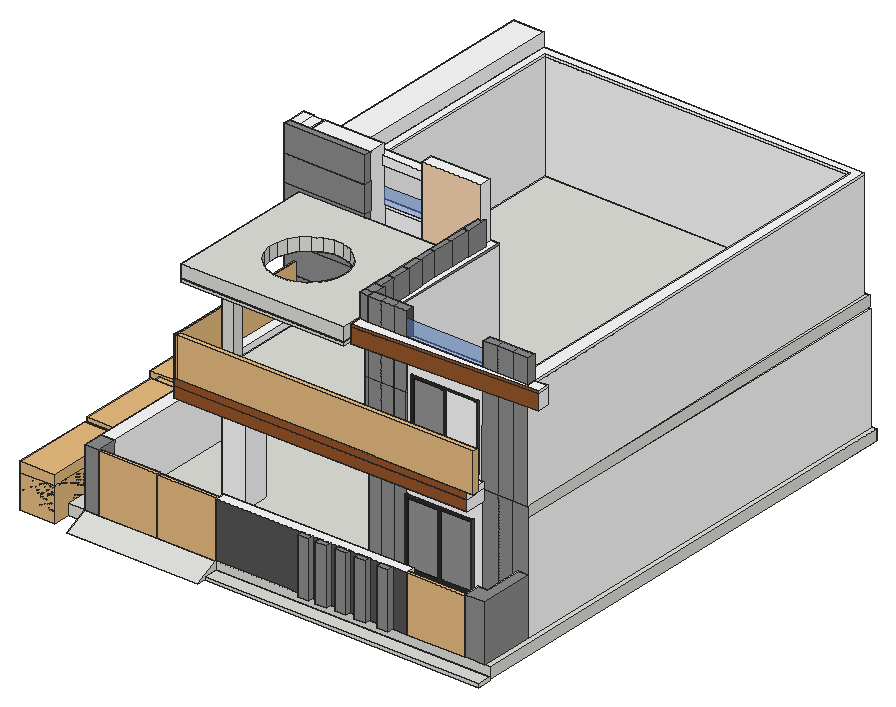
# SketchUp Ruby script. Lengths in inches.
U = 1.inch
M = Sketchup.active_model
def pt(a) = Geom::Point3d.new(a.map { |v| v * U })
def face(e, loops, mat)
  f = e.add_face(loops[0].map { |a| pt(a) })
  loops[1..].each { |l| e.add_face(l.map { |a| pt(a) }).erase! }
  f.material = f.back_material = mat if mat
  f
end
# faces: each face lists its corners as indices into pts; further lists are holes
def faces(e, pts, list, mat = nil) = list.each { |f| face(e, (f[0].is_a?(Array) ? f : [f]).map { |l| l.map { |i| pts[i] } }, mat) }
# xy, xz, yz: faces in a plane at the given z, y or x. An outline is a flat list of corners, or four numbers for a rectangle; further outlines are holes
def ring(l) = l.size == 4 ? [[l[0], l[1]], [l[2], l[1]], [l[2], l[3]], [l[0], l[3]]] : l.each_slice(2).to_a
def flat(e, list, mat, &to3) = list.each { |f| face(e, (f[0].is_a?(Array) ? f : [f]).map { |l| ring(l).map { |u, v| to3.(u, v) } }, mat) }
def xy(e, z, list, mat = nil) = flat(e, list, mat) { |x, y| [x, y, z] }
def xz(e, y, list, mat = nil) = flat(e, list, mat) { |x, z| [x, y, z] }
def yz(e, x, list, mat = nil) = flat(e, list, mat) { |y, z| [x, y, z] }
def lines(e, pts, list) = list.each { |a, b| e.add_line(pt(pts[a]), pt(pts[b])) }
# prism: a flat outline (further loops are holes) pulled along v
def prism(e, loops, v, mat = nil)
  f = face(e, loops, mat); d = Geom::Vector3d.new(v.map { |x| x * U })
  f.pushpull(f.normal.samedirection?(d) ? d.length : -d.length)
end
def box(e, o, s, mat = nil) = prism(e, [[o, [o[0] + s[0], o[1], o[2]], [o[0] + s[0], o[1] + s[1], o[2]], [o[0], o[1] + s[1], o[2]]]], [0, 0, s[2]], mat)
def at(x, y, z, deg = 0) = Geom::Transformation.translation(pt([x, y, z])) * Geom::Transformation.rotation(ORIGIN, Z_AXIS, deg.degrees)
def axes(o, x, y, z) = Geom::Transformation.new([*x, 0, *y, 0, *z, 0, *pt(o).to_a, 1])
def part(name) = M.definitions.add(name)
# library, detail: a bought-in or finely detailed component or shape, given as its bounding box
def library(name, o, s) = part(name).tap { |d| box(d.entities, o, s) }
def detail(e, o, s) = box(e.add_group.entities, o, s)
def put(e, d, t, mat = nil) = e.add_instance(d, t).tap { |i| i.material = mat if mat }
def group(e, t, mat = nil) = e.add_group.tap { |g| g.transformation = t; g.material = mat if mat }.entities
root = M.entities
M.materials.add("Glass_Tinted_Gray").color = [0, 0, 0]
M.materials["Glass_Tinted_Gray"].alpha = 0.125
M.materials.add("[0135_DarkGray]").color = [81, 81, 81]
M.materials.add("[Color C03]").color = [255, 218, 181]
M.materials.add("[Color M00]").color = [255, 255, 255]
M.materials.add("[Color M04]").color = [142, 142, 142]
M.materials.add("[Color M06]").color = [86, 86, 86]
M.materials.add("[Mirror 02]").color = [229, 229, 229]
M.materials.add("[Terrazzo Light Blue]").color = [196, 214, 227]
M.materials.add("[Translucent Glass Blue]").color = [100, 149, 237]
M.materials["[Translucent Glass Blue]"].alpha = 0.5
M.materials.add("[Wood Cherry Original]").color = [152, 86, 42]
c1 = part("PENTEK_RP Fineline 50S_Sliding_DoorCase_E1")
box(c1.entities,[0,0,0],[1.51,3.66,99.27],"[0135_DarkGray]")
c2 = part("PENTEK_RP Fineline 50S_SlidingDooe_Case_E2")
box(c2.entities,[0,0,0],[96.25,3.66,1.51],"[0135_DarkGray]")
c3 = part("pentek_RP Fineline 50S_SlidingDoor_Case")
put(c3.entities,c1,at(97.76,0,0))
put(c3.entities,c2,at(1.51,0,0))
put(c3.entities,c1,at(0,0,0))
put(c3.entities,c2,at(1.51,0,97.76))
c4 = part("PENTEK_RP Fineline 50S_SlidingDoor_GlazingBead_2")
box(c4.entities,[0,0,0],[0.56,0.59,94.39],"[0135_DarkGray]")
c5 = part("PENTEK_RP Fineline 50S_SlidingDoor_Glass")
box(c5.entities,[0,0,0],[46.58,0.16,94.39],"Glass_Tinted_Gray")
c6 = part("PENTEK_RP Fineline 50S_SlidingDoor_GlazingBead")
box(c6.entities,[0,0,0],[45.47,0.59,0.56],"[0135_DarkGray]")
c7 = part("PENTEK_RP Fineline 50S_SlidingDoor_Leaf_E1")
xy(c7.entities,0,[[0,0,0.93,1.97],[0.93,1.57,1.49,1.97]],"[0135_DarkGray]")
xy(c7.entities,96.25,[[0,0,0.93,0,0.93,1.57,1.49,1.57,1.49,1.97,0,1.97]],"[0135_DarkGray]")
xz(c7.entities,0,[[0,0,0.93,96.25]],"[0135_DarkGray]")
xz(c7.entities,1.57,[[0.93,0,1.49,95.32],[0.93,95.32,1.49,96.25]],"[0135_DarkGray]")
xz(c7.entities,1.97,[[0,0,1.49,96.25]],"[0135_DarkGray]")
yz(c7.entities,0,[[0,0,1.97,96.25]],"[0135_DarkGray]")
yz(c7.entities,0.93,[[0,0,1.57,0.93],[0,0.93,1.57,95.32],[0,95.32,1.57,96.25]],"[0135_DarkGray]")
yz(c7.entities,1.49,[[1.57,0,1.97,95.32],[1.57,95.32,1.97,96.25]],"[0135_DarkGray]")
c8 = part("PENTEK_RP Fineline 50S_SlidingDoor_Leaf_E2")
xy(c8.entities,0,[[0,0,0,1.57,0.56,1.57,0.56,1.97,46.02,1.97,46.02,1.57,46.58,1.57,46.58,0]],"[0135_DarkGray]")
xy(c8.entities,0.93,[[0,0,46.58,1.57]],"[0135_DarkGray]")
xy(c8.entities,1.49,[[0.56,1.57,46.02,1.97]],"[0135_DarkGray]")
xz(c8.entities,0,[[0,0,46.58,0.93]],"[0135_DarkGray]")
xz(c8.entities,1.57,[[0,0,0.56,0.93],[46.02,0,46.58,0.93],[0.56,0.93,46.02,1.49]],"[0135_DarkGray]")
xz(c8.entities,1.97,[[0.56,0,46.02,1.49]],"[0135_DarkGray]")
yz(c8.entities,0,[[0,0,1.57,0.93]],"[0135_DarkGray]")
yz(c8.entities,0.56,[[1.57,0,1.97,0.93],[1.57,0.93,1.97,1.49]],"[0135_DarkGray]")
yz(c8.entities,46.02,[[1.57,0,1.97,0.93],[1.57,0.93,1.97,1.49]],"[0135_DarkGray]")
yz(c8.entities,46.58,[[0,0,1.57,0.93]],"[0135_DarkGray]")
c9 = part("PENTEK_RP Fineline S_SlidingDoor_Leaf1")
put(c9.entities,c4,at(0.93,0,0.93))
put(c9.entities,c4,at(46.96,0,0.93))
put(c9.entities,c5,at(1.49,1.42,0.93))
put(c9.entities,c6,at(1.49,0,0.93))
put(c9.entities,c5,at(1.49,0.59,0.93),"[Terrazzo Light Blue]")
put(c9.entities,c7,at(0,0,0))
put(c9.entities,c7,axes([48.44,0,0],[-1,0,0],[0,1,0],[0,0,1]))
put(c9.entities,c8,axes([0.93,0,96.25],[1,0,0],[0,1,0],[0,0,-1]))
put(c9.entities,c8,at(0.93,0,0))
put(c9.entities,c6,at(1.49,0,94.77))
c10 = part("PENTEK_RP Fineline 50S_SlidingDoor_Leaf2")
put(c10.entities,c5,at(1.49,1.42,0.93))
put(c10.entities,c6,at(1.49,0,94.77))
put(c10.entities,c4,at(46.96,0,0.93))
put(c10.entities,c5,at(1.49,0.59,0.93),"[Mirror 02]")
put(c10.entities,c4,at(0.93,0,0.93))
put(c10.entities,c7,at(0,0,0))
put(c10.entities,c7,axes([48.44,0,0],[-1,0,0],[0,1,0],[0,0,1]))
put(c10.entities,c6,at(1.49,0,0.93))
put(c10.entities,c8,axes([0.93,0,96.25],[1,0,0],[0,1,0],[0,0,-1]))
put(c10.entities,c8,at(0.93,0,0))
c11 = part("PENTEK - Slimmest Steel Sliding Door / Window\#1")
put(c11.entities,c3,at(0,-1.88,-0.09))
put(c11.entities,c9,at(1.51,-2.27,1.42))
put(c11.entities,c10,at(49.32,-0.3,1.42))
c12 = library("door",[38.93,25.48,0],[40,9.94,82.68])
c13 = library("4",[-16.3,-15.81,0],[32.6,31.62,37.8])
c14 = library("Glass railing",[-3.84,-0.8125,0],[184.69,5.8,43.77])
c15 = library("GATE",[0,0,0],[65.3125,3.71,50.96])
c16 = library("Broadleaf shrub",[-20.25,-26.94,0.18],[38.61,38.31,37.53])
box(root,[161.95,100.9375,132],[13.31,11.6875,105.125])
xy(root,-12,[[68.78,0,215.96,24.87],[215.96,8.81,523.46,24.87]])
xy(root,-8.5,[[215.96,8.81,523.46,24.87]])
xy(root,-0.5,[[151.43,114.08,151.27,142.08,178.52,142.08,178.52,114.08]],"[Color M00]")
xy(root,0,[[68.78,24.89,84.94,47.54],[215.5625,25.71,399.99,26.76,412.56,26.83,428.17,26.92,428.11,37.92,215.5,36.71],[493.76,27.36,493.76,45.88,504.01,45.88,504.01,88.97,515.68,89.71,515.68,27.36],[68.78,47.54,84.94,47.54,84.94,542.67,155.68,542.67,155.68,569.71,68.78,569.71],[504.01,88.97,515.68,89.71,504.01,89.71],
  [[335.68,89.71,335.68,261.83,155.68,261.83,155.68,569.71,515.68,569.71,515.68,89.71],[344.68,98.71,506.68,98.71,506.68,560.71,164.68,560.71,164.68,270.83,344.68,270.83]],[344.68,98.71,506.68,98.71,506.68,560.71,164.68,560.71,164.68,270.83,344.68,270.83]],"[Color M00]")
xy(root,62.34,[[215.5625,25.71,215.5,36.71,428.11,37.92,428.17,26.92,412.56,26.83,399.99,26.76]],"[Color M00]")
xy(root,63.0625,[[493.76,27.36,515.68,27.36,515.68,89.71,504.01,88.97,504.01,45.88,493.76,45.88]],"[Color M04]")
xy(root,65.5625,[[68.78,47.54,68.78,569.71,155.68,569.71,155.68,542.67,84.94,542.67,84.94,47.54]],"[Color M00]")
xy(root,65.5625,[[68.78,24.89,84.94,47.54]],"[Color M04]")
xy(root,73.4375,[[125.21,233.58,136.89,241.14],[136.93,233.58,136.89,241.14,136.8,257.14,212.86,257.58,212.99,234.01],[125.64,241.14,125.64,260.77,136.78,260.77,136.8,257.14,136.89,241.14]],"[Color M00]")
xy(root,97.01,[[136.8,257.14,136.8,257.39,212.86,257.83,212.86,257.58]],"[Color M00]")
xy(root,119.3125,[[114.96,260.97,148.83,568.64]],"[Color M00]")
xy(root,120,[[137.9,63.43,136.93,233.58,150.74,233.66,151.27,142.08,151.27,114.08,151.43,114.08,151.58,87.63,335.96,88.68,339.22,88.7,364.71,88.85,376.84,88.92,378.17,88.92,465.72,89.42,465.86,65.3],[[335.68,89.71,515.68,89.71,515.68,569.71,155.68,569.71,155.68,261.83,335.68,261.83],[344.68,98.71,344.68,270.83,164.68,270.83,164.68,560.71,506.68,560.71,506.68,98.71]],[151.27,114.08,151.27,142.08,151.43,114.08],[151.43,114.08,178.52,114.08,178.52,142.08,151.27,142.08],[150.74,233.66,212.99,234.01,212.86,257.83,150.61,257.47],
  [136.8,257.39,136.78,260.77,136.77,261.05,150.59,261.13,150.61,257.47]],"[Color M00]")
xy(root,131.4375,[[337.83,97.64,499.83,97.64,499.83,559.64,157.83,559.64,157.83,269.77,337.83,269.77]],"[Color M00]")
xy(root,132,[[137.9,63.43,465.86,65.3,465.72,88.64,335.96,88.64,332.77,88.51,332.77,88.66,151.58,87.63,150.7,241.14,136.89,241.14],[332.77,88.51,332.77,88.66,364.71,88.85,465.72,89.42,465.72,89.38,378.17,88.88,339.22,88.66,335.96,88.64],[[465.72,88.64,465.72,89.42,364.71,88.85,332.77,88.66,332.1875,102.6,335.375,102.73,328.83,260.77,216.72,260.77,216.72,241.14,150.7,241.14,150.59,260.77,150.59,261.13,148.83,261.12,148.83,568.64,508.83,568.64,515.57,89.7,498.73,88.64],[337.83,97.64,499.83,97.64,499.83,559.64,157.83,559.64,157.83,269.77,337.83,269.77]],[335.96,88.64,339.22,88.66,378.17,88.88,465.72,89.38,465.72,89.36,339.22,88.64],[339.22,88.64,465.72,89.36,465.72,88.79,439.91,88.64],
  [439.91,88.64,465.72,88.79,465.72,88.64],[498.73,88.64,515.57,89.7,515.58,88.64],[136.89,241.14,136.89,260.77,136.78,260.77],[136.89,241.14,148.96,260.77],[148.96,241.14,150.34,260.77],
  [150.34,241.14,150.7,241.14,150.59,260.77,150.34,260.77],[263.14,255.33,270.72,260.77],[310.72,255.33,328.83,260.77],[136.78,260.77,148.83,260.77,148.83,260.97,136.77,260.97],[148.83,260.77,148.83,261.12,150.59,261.13,150.59,260.77],
  [136.77,260.97,148.83,260.97,148.83,261.12,136.77,261.05],[114.96,285.03,131.08,285.03,131.89,553.28,114.96,553.28],[131.08,285.03,148.83,285.03,148.83,553.28,131.89,553.28]],"[Color M00]")
xy(root,139.01,[[125.21,233.58,136.89,241.14]],"[Color M00]")
xy(root,139.5625,[[137.9,63.43,465.86,65.3,465.72,88.64,335.96,88.64,332.77,88.51,332.77,88.66,151.58,87.63,150.59,260.77,148.83,260.77,148.83,261.12,136.77,261.05,136.77,260.97,136.89,241.14]],"[Color M00]")
xy(root,225.26,[[270.72,255.33,310.72,260.77]],"[Color M00]")
xy(root,230.5625,[[114.96,285.03,148.83,553.28]],"[Color M00]")
xy(root,235.0625,[[326.7,76.5,319.09,260.36,328.83,260.77,335.375,102.73,332.1875,102.6,332.77,88.51,335.96,88.64,515.48,96.07,515.41,97.64,529.98,98.24,530.53,84.9375]],"[Color M00]")
xy(root,240.21,[[[142.34,68.02,324.65,233.58],[229.57,102.99,239.9375,105.52,249.29,110.64,257.01,118.01,262.55,127.13,265.55,137.37,265.79,148.04,263.26,158.41,258.13,167.77,250.76,175.48,241.64,181.02,231.4,184.02,220.73,184.26,210.37,181.73,201.01,176.61,193.29,169.23,187.75,160.12,184.76,149.875,184.52,139.21,187.04,128.84,192.17,119.48,199.54,111.77,208.66,106.22,218.9,103.23]]])
xy(root,252,[[326.7,76.5,319.09,260.36,328.83,260.77,148.83,260.77,148.83,568.64,508.83,568.64,515.46,97.64,499.83,97.64,499.83,559.64,157.83,559.64,157.83,269.77,337.83,269.77,337.83,97.64,335.58,97.64,335.96,88.64,378.93,90.42,378.93,88.64,465.05,88.64,465.05,93.99,515.48,96.07,515.41,97.64,515.46,97.64,529.98,98.24,530.53,84.9375],[378.93,88.64,465.05,88.64,465.05,93.99,378.93,90.42],[378.93,90.42,465.05,93.99,465.05,97.64,378.93,97.64]],"[Color M00]")
xy(root,254.34,[[[142.34,68.02,324.65,233.58],[229.57,102.99,218.9,103.23,208.66,106.22,199.54,111.77,192.17,119.48,187.04,128.84,184.52,139.21,184.76,149.875,187.75,160.12,193.29,169.23,201.01,176.61,210.37,181.73,220.73,184.26,231.4,184.02,241.64,181.02,250.76,175.48,258.13,167.77,263.26,158.41,265.79,148.04,265.55,137.37,262.55,127.13,257.01,118.01,249.29,110.64,239.9375,105.52]]])
xy(root,254.875,[[326.7,76.5,530.53,84.9375,529.98,98.24,515.46,97.64,515.48,96.07,465.05,93.99,465.05,88.64,378.93,88.64,378.93,90.42,335.96,88.64,335.66,95.79,335.58,97.64,335.58,95.79,335.66,95.79,335.66,88.64,326.2,88.64,326.2,109.3,325.34,109.3,326.2,88.64],[515.48,96.07,515.46,97.64,515.41,97.64],[[499.83,97.64,515.46,97.64,508.83,568.64,148.83,568.64,148.83,260.77,263.14,260.77,263.14,268.2,328.83,268.2,328.83,260.77,319.09,260.36,325.34,109.3,326.2,109.3,326.2,127.73,326.5,127.73,326.5,148.09,333.9375,148.09,333.9375,127.73,333.88,127.73,333.88,109.3,337.83,109.3,337.83,269.77,157.83,269.77,157.83,559.64,499.83,559.64],[325.7,167.61,325.7,210.94,325.6,210.94,325.6,234.09,325.43,234.09,325.43,258.07,332.24,258.07,332.24,234.09,331.91,234.09,331.91,210.94,332.06,210.94,332.06,187.3125,331.56,187.3125,331.56,167.61],[326.5,148.09,325.7,167.37,331.56,167.61,333.08,167.67,333.875,148.4]],[136.89,260.27,148.96,260.77],[150.34,260.27,216.72,260.77],
  [216.72,260.27,263.14,260.77,216.72,260.77],[263.14,260.77,328.83,268.2],[114.96,553.28,148.83,568.64]],"[Color M00]")
xy(root,269.75,[[114.96,260.97,136.77,260.97,136.77,261.05,148.83,261.12,148.83,568.64,114.96,568.64]],"[Color M00]")
xy(root,281.3125,[[326.2,88.64,335.66,95.79],[335.96,88.64,350.49,88.64,350.49,97.64,335.58,97.64,335.66,95.79],[350.49,88.64,364.71,97.64],[364.71,88.64,378.93,97.64],[465.05,88.64,480.99,97.64],
  [480.99,88.64,498.29,97.64],[498.29,88.64,515.58,88.64,515.46,97.64,498.29,97.64],[326.2,95.79,335.58,95.79,335.58,97.64,337.83,97.64,337.83,109.3,326.2,109.3],[326.2,109.3,333.88,127.73],[326.5,127.73,333.9375,148.09],
  [326.5,148.09,333.875,148.4,333.08,167.67,331.56,167.61,325.7,167.37],[325.7,167.61,331.56,187.3125],[325.7,187.3125,332.06,210.94],[325.6,210.94,331.91,234.09],[325.43,234.09,332.24,258.07]],"[Color M04]")
xy(root,297.05,[[216.72,256.41,216.72,260.27,212.1,260.27,212.1,266.91,263.14,266.91,263.14,256.41]],"[Color M00]")
xy(root,306.86,[[216.72,256.41,263.14,256.41,263.14,266.91,212.1,266.91,212.1,260.27,216.72,260.27]],"[Color M00]")
xy(root,317.125,[[125.64,241.14,136.89,260.77],[136.89,241.14,148.96,260.27],[150.34,241.14,216.72,260.27],[263.14,255.33,328.83,268.2]],"[Color M00]")
xz(root,8.81,[[215.96,-12,523.46,-8.5]])
xz(root,24.87,[[215.96,-12,523.46,-8.5]])
xz(root,24.89,[[68.78,0,84.94,65.5625]],"[Color M04]")
xz(root,27.36,[[493.76,0,515.68,63.0625]],"[Color M04]")
xz(root,45.88,[[493.76,0,504.01,63.0625]],"[Color M00]")
xz(root,47.54,[[68.78,0,84.94,65.5625]],"[Color M00]")
xz(root,68.02,[[142.34,235.59,324.65,238.96],[142.34,238.96,324.65,240.21],[142.34,240.21,324.65,254.34]])
xz(root,88.64,[[335.96,132,339.22,139.5625],[339.22,132,350.49,139.5625],[350.49,132,364.71,139.5625],[364.71,132,378.93,139.5625],[378.93,132,439.91,139.5625],
  [439.91,132,463.57,139.5625],[463.57,132,463.66,139.5625,463.57,139.5625],[378.93,139.5625,463.66,139.5625,465.05,252,378.93,252],[378.93,252,465.05,254.875]],"[Color M00]")
xz(root,88.64,[[465.72,132,481.89,132,480.99,252,465.05,252,463.66,139.5625,465.72,139.5625],[481.89,132,498.73,132,498.29,252,480.99,252],[498.73,132,515.58,132,515.58,281.3125,498.29,281.3125,498.29,252],[335.96,139.5625,350.49,281.3125],[350.49,139.5625,378.93,139.5625,378.93,252,364.71,252,364.71,281.3125,350.49,281.3125],
  [364.71,252,378.93,281.3125],[465.05,252,480.99,281.3125],[480.99,252,498.29,281.3125],[326.2,254.875,335.66,281.3125]],"[Color M04]")
xz(root,88.64,[[463.57,132,463.66,139.5625,465.72,139.5625,465.72,132]],"[Color M06]")
xz(root,88.64,[[378.93,254.875,465.05,274.03]],"[Translucent Glass Blue]")
xz(root,89.71,[[335.68,0,515.68,120]],"[Color M04]")
xz(root,95.79,[[335.58,254.875,335.66,281.3125]],"[Color M00]")
xz(root,97.64,[[337.83,131.4375,499.83,132],[335.58,252,337.83,254.875],[499.83,252,515.46,254.875],[515.41,252,515.46,254.875],[335.58,254.875,337.83,281.3125],
  [499.83,254.875,515.46,281.3125]],"[Color M00]")
xz(root,97.64,[[337.83,132,337.83,281.3125,378.93,281.3125,378.93,252,465.05,252,465.05,281.3125,499.83,281.3125,499.83,132]],"[Color M04]")
xz(root,98.71,[[344.68,0,506.68,120]],"[Color M00]")
xz(root,109.3,[[326.2,254.875,333.88,281.3125],[333.88,254.875,337.83,281.3125]],"[Color M00]")
xz(root,114.08,[[151.43,-0.5,178.52,120]],"[Color M00]")
xz(root,127.73,[[326.2,254.875,326.5,281.3125],[326.5,254.875,333.88,281.3125],[333.88,254.875,333.9375,281.3125]],"[Color M00]")
xz(root,142.08,[[151.27,-0.5,178.52,120]],"[Color M00]")
xz(root,148.09,[[326.5,254.875,333.9375,281.3125]],"[Color M00]")
xz(root,167.61,[[325.7,254.875,331.56,281.3125]],"[Color M00]")
xz(root,187.3125,[[325.7,254.875,331.56,281.3125]],"[Color M00]")
xz(root,210.94,[[325.6,254.875,325.7,281.3125],[325.7,254.875,331.91,281.3125],[331.91,254.875,332.06,281.3125]],"[Color M00]")
xz(root,233.58,[[142.34,235.59,324.65,238.96],[142.34,238.96,324.65,240.21],[142.34,240.21,324.65,254.34]])
xz(root,233.58,[[136.89,97.01,136.93,120],[136.89,97.01,136.93,120]],"[Color M00]")
xz(root,233.58,[[125.21,73.4375,136.89,97.01],[125.21,97.01,136.89,120],[125.21,120,136.89,139.01]],"[Color M04]")
xz(root,234.09,[[325.43,254.875,325.6,281.3125],[325.6,254.875,331.91,281.3125],[331.91,254.875,332.24,281.3125]],"[Color M00]")
xz(root,241.14,[[125.21,73.4375,125.64,139.01],[136.89,132,148.96,132,148.96,287.4375,136.89,287.4375,136.89,317.125,125.64,317.125,125.64,139.01,136.89,139.01],[150.34,132,216.72,287.4375],[136.89,287.4375,148.96,317.125],[148.96,287.4375,150.34,317.125]],"[Color M00]")
xz(root,255.33,[[263.14,132,270.72,132,270.72,225.26,310.72,225.26,310.72,132,328.83,132,328.83,317.125,263.14,317.125]],"[Color C03]")
xz(root,256.41,[[216.72,297.05,263.14,306.86]],"[Color M00]")
xz(root,258.07,[[325.43,254.875,332.24,281.3125]],"[Color M06]")
xz(root,260.27,[[136.89,254.875,148.96,317.125],[150.34,254.875,216.72,254.875,216.72,297.05,212.1,297.05,212.1,306.86,216.72,306.86,216.72,317.125,150.34,317.125],[212.1,297.05,216.72,306.86]],"[Color M00]")
xz(root,260.77,[[125.64,73.4375,125.64,317.125,136.89,317.125,136.89,252,148.83,252,148.83,139.5625,136.89,139.5625,136.89,132,136.78,132,136.78,73.4375],[136.89,132,148.83,139.5625],[148.83,132,148.96,139.5625],[148.96,132,150.34,139.5625],[150.34,132,150.59,139.5625],
  [216.72,132,263.14,252],[270.72,132,310.72,225.26],[148.83,139.5625,148.96,252],[148.96,139.5625,150.34,252],[136.89,252,148.83,254.875],
  [148.83,252,148.96,254.875],[148.96,252,150.34,254.875],[150.34,252,216.72,254.875],[216.72,252,263.14,254.875],[263.14,252,328.83,254.875]],"[Color M00]")
xz(root,260.97,[[114.96,119.3125,148.83,119.3125,148.83,132,136.77,132,136.77,269.75,114.96,269.75]],"[Wood Cherry Original]")
xz(root,261.83,[[155.68,0,335.68,120]],"[Color M00]")
xz(root,266.91,[[212.1,297.05,263.14,306.86]],"[Color M00]")
xz(root,268.2,[[263.14,254.875,328.83,317.125]],"[Color M00]")
xz(root,269.77,[[157.83,131.4375,337.83,132],[157.83,132,337.83,252],[157.83,252,337.83,254.875]],"[Color M00]")
xz(root,270.83,[[164.68,0,344.68,120]],"[Color M00]")
xz(root,285.03,[[114.96,132,148.83,230.5625]],"[Color M00]")
xz(root,542.67,[[84.94,0,155.68,65.5625]],"[Color M00]")
xz(root,553.28,[[114.96,132,148.83,230.5625],[114.96,230.5625,148.83,254.875]],"[Color M00]")
xz(root,559.64,[[157.83,131.4375,499.83,132],[157.83,132,499.83,252],[157.83,252,499.83,254.875]],"[Color M00]")
xz(root,560.71,[[164.68,0,506.68,120]],"[Color M00]")
xz(root,568.64,[[114.96,119.3125,148.83,254.875],[148.83,132,508.83,252],[148.83,252,508.83,254.875],[114.96,254.875,148.83,269.75]],"[Color M00]")
xz(root,569.71,[[68.78,0,155.68,65.5625],[155.68,0,515.68,120]],"[Color M00]")
yz(root,68.78,[[0,-12,24.89,0,24.87,-12]])
yz(root,68.78,[[47.54,0,569.71,65.5625]],"[Color M00]")
yz(root,68.78,[[24.89,0,47.54,65.5625]],"[Color M04]")
yz(root,84.94,[[47.54,0,542.67,65.5625]],"[Color M00]")
yz(root,84.94,[[24.89,0,47.54,65.5625]],"[Color M04]")
yz(root,114.96,[[[260.97,119.3125,568.64,269.75],[285.03,132,553.28,230.5625]]],"[Wood Cherry Original]")
yz(root,125.21,[[233.58,73.4375,241.14,139.01]],"[Color M04]")
yz(root,125.64,[[241.14,73.4375,260.77,317.125]],"[Color C03]")
yz(root,136.77,[[260.97,132,261.05,139.5625],[260.97,139.5625,261.05,269.75]],"[Color M00]")
yz(root,136.89,[[233.58,73.4375,241.14,139.01],[260.27,254.875,260.77,317.125]],"[Color M00]")
yz(root,142.34,[[68.02,235.59,233.58,238.96],[68.02,238.96,233.58,240.21],[68.02,240.21,233.58,254.34]])
yz(root,148.83,[[260.97,119.3125,568.64,132],[260.77,132,261.12,139.5625],[261.12,132,285.03,252],[285.03,132,553.28,230.5625],[260.77,139.5625,261.12,252],
  [285.03,230.5625,553.28,252],[260.77,252,261.12,254.875],[261.12,252,285.03,254.875],[285.03,252,553.28,254.875],[553.28,252,568.64,254.875],
  [261.12,254.875,568.64,269.75]],"[Color M00]")
yz(root,148.96,[[241.14,132,260.77,132,260.77,254.875,260.27,254.875,260.27,317.125,241.14,317.125]],"[Color M00]")
yz(root,150.34,[[241.14,132,260.77,132,260.77,254.875,260.27,254.875,260.27,317.125,241.14,317.125]],"[Color M00]")
yz(root,155.68,[[261.83,0,261.83,120,569.71,120,569.71,65.5625,542.67,65.5625,542.67,0],[542.67,0,569.71,65.5625]],"[Color M00]")
yz(root,157.83,[[269.77,131.4375,559.64,132],[269.77,132,559.64,252],[269.77,252,559.64,254.875]],"[Color M00]")
yz(root,164.68,[[270.83,0,560.71,120]],"[Color M00]")
yz(root,178.52,[[114.08,-0.5,142.08,120]],"[Color M00]")
yz(root,212.1,[[260.27,297.05,266.91,306.86]],"[Color M00]")
yz(root,215.96,[[0,-12,8.81,-12,8.81,-8.5,24.87,-8.5,24.87,-12,24.89,0],[8.81,-12,24.87,-8.5]])
yz(root,216.72,[[241.14,132,260.77,132,260.77,254.875,260.27,254.875,260.27,297.05,256.41,297.05,256.41,306.86,260.27,306.86,260.27,317.125,241.14,317.125],[256.41,297.05,260.27,306.86]],"[Color M00]")
yz(root,263.14,[[[255.33,132,255.33,317.125,268.2,317.125,268.2,274.34,260.77,274.34,260.77,132],[256.41,297.05,266.91,306.86]]],"[Color C03]")
yz(root,263.14,[[260.77,254.875,268.2,274.34]],"[Color M00]")
yz(root,270.72,[[255.33,132,260.77,225.26]],"[Color M00]")
yz(root,310.72,[[255.33,132,260.77,225.26]],"[Color M00]")
yz(root,324.65,[[68.02,235.59,233.58,238.96],[68.02,238.96,233.58,240.21],[68.02,240.21,233.58,254.34]])
yz(root,325.43,[[234.09,254.875,258.07,281.3125]],"[Color M04]")
yz(root,325.6,[[210.94,254.875,234.09,281.3125]],"[Color M04]")
yz(root,325.7,[[167.61,254.875,187.3125,281.3125],[187.3125,254.875,210.94,281.3125]],"[Color M04]")
yz(root,326.2,[[88.64,254.875,95.79,281.3125],[95.79,254.875,109.3,281.3125],[109.3,254.875,127.73,281.3125]],"[Color M04]")
yz(root,326.5,[[127.73,254.875,148.09,281.3125]],"[Color M04]")
yz(root,328.83,[[255.33,132,260.77,132,260.77,254.875,268.2,254.875,268.2,317.125,255.33,317.125]],"[Color M00]")
yz(root,331.56,[[167.61,254.875,187.3125,281.3125]],"[Color M04]")
yz(root,331.91,[[210.94,254.875,234.09,281.3125]],"[Color M04]")
yz(root,332.06,[[187.3125,254.875,210.94,281.3125]],"[Color M04]")
yz(root,332.24,[[234.09,254.875,258.07,281.3125]],"[Color M04]")
yz(root,332.77,[[88.51,132,88.66,139.5625]],"[Color M00]")
yz(root,333.88,[[109.3,254.875,127.73,281.3125]],"[Color M04]")
yz(root,333.9375,[[127.73,254.875,148.09,281.3125]],"[Color M04]")
yz(root,335.58,[[95.79,254.875,97.64,281.3125]],"[Color M00]")
yz(root,335.66,[[88.64,254.875,95.79,281.3125]],"[Color M00]")
yz(root,335.68,[[89.71,0,261.83,120]],"[Color M00]")
yz(root,337.83,[[97.64,131.4375,269.77,132],[97.64,132,269.77,252]],"[Color M00]")
yz(root,337.83,[[97.64,252,269.77,252,269.77,254.875,109.3,254.875,109.3,281.3125,97.64,281.3125]],"[Color M04]")
yz(root,344.68,[[98.71,0,270.83,120]],"[Color M00]")
yz(root,364.71,[[88.85,203.61,88.79,216.16,88.85,245.625]],"[Color M00]")
yz(root,378.93,[[88.64,252,90.42,254.875]],"[Color M00]")
yz(root,378.93,[[90.42,252,97.64,252,97.64,281.3125,88.64,281.3125,88.64,254.875,90.42,254.875]],"[Color M06]")
yz(root,465.05,[[88.64,252,93.99,254.875]],"[Color M00]")
yz(root,465.05,[[93.99,252,93.99,254.875,88.64,254.875,88.64,281.3125,97.64,281.3125,97.64,252]],"[Color M04]")
yz(root,493.76,[[27.36,0,45.88,63.0625]],"[Color M00]")
yz(root,499.83,[[97.64,131.4375,559.64,132],[97.64,132,559.64,252],[97.64,252,559.64,254.875]],"[Color M00]")
yz(root,504.01,[[45.88,0,88.97,63.0625]],"[Color M00]")
yz(root,506.68,[[98.71,0,560.71,120]],"[Color M00]")
yz(root,515.68,[[89.71,0,569.71,120]],"[Color M00]")
yz(root,515.68,[[27.36,0,89.71,63.0625]],"[Color M04]")
yz(root,523.46,[[8.81,-12,24.87,-8.5]])
p = [[68.78,24.89,0],[68.78,0,-12],[215.96,0,-12],[215.96,24.89,0],[84.94,24.89,0],[68.78,24.87,-12],
  [215.96,24.87,-12],[151.43,114.08,120],[151.27,142.08,120],[151.27,142.08,-0.5],[151.43,114.08,-0.5],[215.5625,25.71,0],
  [215.5,36.71,0],[215.5,36.71,62.34],[215.5625,25.71,62.34],[399.99,26.76,62.34],[399.99,26.76,0],[428.17,26.92,0],
  [412.56,26.83,0],[412.56,26.83,62.34],[428.17,26.92,62.34],[428.11,37.92,0],[428.11,37.92,62.34],[364.71,88.64,252],
  [364.71,88.79,216.16],[364.71,88.85,203.61],[364.71,89.71,0],[376.84,89.71,0],[378.93,88.64,252],[463.57,89.71,0],
  [465.05,88.64,252],[481.89,89.71,0],[480.99,88.64,252],[498.79,89.71,0],[498.29,88.64,252],[515.57,89.7,132],
  [498.73,88.64,132],[498.73,88.64,0],[504.01,88.97,0],[504.01,88.97,63.0625],[515.68,89.71,63.0625],[515.68,89.71,120],
  [515.68,89.71,132],[515.68,89.71,0],[136.93,233.58,97.01],[136.89,241.14,97.01],[136.89,241.14,73.4375],[136.93,233.58,73.4375],
  [212.99,234.01,73.4375],[212.99,234.01,97.01],[212.86,257.58,97.01],[212.86,257.58,73.4375],[136.8,257.14,73.4375],[136.8,257.14,97.01],
  [136.78,260.77,73.4375],[136.78,260.77,120],[136.8,257.39,120],[136.8,257.39,97.01],[136.93,233.58,120],[212.99,234.01,120],
  [150.74,233.66,120],[136.89,241.14,120],[212.86,257.83,120],[212.86,257.83,97.01],[150.61,257.47,120],[137.9,63.43,132],
  [136.89,241.14,132],[137.9,63.43,120],[465.86,65.3,120],[465.86,65.3,132],[465.72,89.42,120],[465.72,89.42,132],
  [465.72,89.38,132],[465.72,89.36,132],[465.72,88.79,132],[465.72,88.64,132],[151.58,87.63,132],[151.58,87.63,120],
  [150.59,261.13,120],[150.59,261.13,132],[150.59,260.77,132],[150.7,241.14,132],[335.96,88.68,120],[332.77,88.66,132],
  [364.71,88.85,132],[364.71,88.85,120],[339.22,88.7,120],[339.22,88.66,132],[335.96,88.64,132],[376.84,88.92,120],
  [378.17,88.92,120],[378.17,88.88,132],[136.78,260.77,132],[136.77,261.05,120],[136.77,260.97,132],[136.77,261.05,132],
  [148.83,261.12,132],[137.9,63.43,139.5625],[136.89,241.14,139.5625],[136.89,241.14,139.01],[465.86,65.3,139.5625],[465.72,88.64,139.5625],
  [150.59,260.77,139.5625],[151.58,87.63,139.5625],[332.77,88.66,139.5625],[332.77,88.51,139.5625],[332.77,88.51,199],[332.1875,102.6,199],
  [332.1875,102.6,132],[332.77,88.51,132],[335.96,88.64,139.5625],[515.46,97.64,252],[515.46,97.64,254.875],[515.48,96.07,254.875],
  [515.58,88.64,254.875],[515.58,88.64,132],[508.83,568.64,132],[508.83,568.64,252],[335.375,102.73,235.0625],[335.375,102.73,132],
  [332.1875,102.6,235.0625],[328.83,260.77,132],[328.83,260.77,235.0625],[136.77,260.97,139.5625],[136.77,261.05,139.5625],[148.83,261.12,139.5625],
  [131.89,553.8,132],[131.89,553.28,132],[131.08,285.03,132],[131.08,285.03,164.86],[131.89,553.8,164.86],[335.96,88.64,235.0625],
  [332.77,88.51,235.0625],[148.83,261.12,252],[148.83,261.12,254.875],[148.83,261.12,269.75],[136.77,261.05,269.75],[319.09,260.36,252],
  [319.09,260.36,235.0625],[326.7,76.5,235.0625],[326.7,76.5,252],[530.53,84.9375,235.0625],[530.53,84.9375,252],[529.98,98.24,235.0625],
  [529.98,98.24,252],[465.05,93.99,252],[515.48,96.07,252],[515.48,96.07,235.0625],[335.96,88.64,252],[378.93,90.42,252],
  [515.41,97.64,252],[515.41,97.64,235.0625],[328.83,260.77,252],[218.9,103.23,254.34],[229.57,102.99,254.34],[229.57,102.99,240.21],
  [218.9,103.23,240.21],[239.9375,105.52,254.34],[239.9375,105.52,240.21],[208.66,106.22,254.34],[208.66,106.22,240.21],[249.29,110.64,254.34],
  [249.29,110.64,240.21],[199.54,111.77,254.34],[199.54,111.77,240.21],[257.01,118.01,254.34],[257.01,118.01,240.21],[192.17,119.48,254.34],
  [192.17,119.48,240.21],[262.55,127.13,254.34],[262.55,127.13,240.21],[187.04,128.84,254.34],[187.04,128.84,240.21],[265.55,137.37,254.34],
  [265.55,137.37,240.21],[184.52,139.21,254.34],[184.52,139.21,240.21],[265.79,148.04,254.34],[265.79,148.04,240.21],[184.76,149.875,254.34],
  [184.76,149.875,240.21],[263.26,158.41,254.34],[263.26,158.41,240.21],[187.75,160.12,254.34],[187.75,160.12,240.21],[258.13,167.77,254.34],
  [258.13,167.77,240.21],[193.29,169.23,254.34],[193.29,169.23,240.21],[250.76,175.48,254.34],[250.76,175.48,240.21],[201.01,176.61,254.34],
  [201.01,176.61,240.21],[241.64,181.02,254.34],[241.64,181.02,240.21],[210.37,181.73,254.34],[210.37,181.73,240.21],[231.4,184.02,254.34],
  [231.4,184.02,240.21],[220.73,184.26,254.34],[220.73,184.26,240.21],[326.7,76.5,254.875],[326.2,88.64,254.875],[325.34,109.3,254.875],
  [319.09,260.36,254.875],[530.53,84.9375,254.875],[529.98,98.24,254.875],[335.58,97.64,252],[335.96,88.64,254.875],[335.66,95.79,254.875],
  [335.58,97.64,254.875],[378.93,90.42,254.875],[465.05,93.99,254.875],[515.41,97.64,254.875],[508.83,568.64,254.875],[328.83,260.77,254.875],
  [335.96,88.64,281.3125],[335.66,95.79,281.3125],[515.58,88.64,281.3125],[515.46,97.64,281.3125],[335.58,97.64,281.3125],[325.7,167.37,254.875],
  [326.5,148.09,254.875],[326.5,148.09,281.3125],[325.7,167.37,281.3125],[333.875,148.4,254.875],[333.875,148.4,281.3125],[333.08,167.67,254.875],
  [333.08,167.67,281.3125],[331.56,167.61,281.3125],[331.56,167.61,254.875],[263.14,260.77,254.875],[216.72,260.27,254.875],[216.72,260.27,274.34],
  [263.14,260.77,274.34],[350.49,88.64,132],[350.49,88.64,0],[364.71,88.64,132],[364.71,88.64,139.5625],[364.71,88.64,245.625],
  [148.96,260.27,317.125],[150.34,260.27,317.125],[148.96,260.27,254.875],[150.34,260.27,254.875],[378.33,88.51,199]]
faces(root,p,[[0,1,2,3,4],[5,0,4,3,6],[153,154,155,156],[154,157,158,155],[159,153,156,160],[157,161,162,158],[163,159,160,164],[161,165,166,162],
  [167,163,164,168],[165,169,170,166],[171,167,168,172],[169,173,174,170],[175,171,172,176],[173,177,178,174],[179,175,176,180],[177,181,182,178],
  [183,179,180,184],[181,185,186,182],[187,183,184,188],[185,189,190,186],[191,187,188,192],[189,193,194,190],[195,191,192,196],[193,197,198,194],
  [199,195,196,200],[197,199,200,198]])
faces(root,p,[[7,8,9,10],[11,12,13,14],[21,17,20,22],[12,21,22,13],[28,27,29,30],[38,43,40,39],[44,45,46,47],[50,49,48,51],
  [52,53,50,51],[53,52,54,55,56,57],[61,45,44,58],[62,59,49,50,63],[57,56,64,62,63],[70,71,72,73,74,75,69,68],[76,77,7,8,60,64,78,79,80,81],[82,77,76,83,84,85,86],
  [89,85,84,71,70,90],[55,56,61,66,92],[93,55,92,94,95],[96,79,78,93,95],[69,75,101,100],[76,81,80,102,103],[83,76,103,104],[109,88,110,105],
  [111,112,113,114,115,35,116,117],[118,119,108,107,120],[121,119,118,122],[98,123,94,92,66,99],[96,95,124,125],[124,125,133,134,135,136],[141,143,144,142],[145,146,147,131,148,149],
  [147,146,150,151],[143,151,150,111,144],[152,122,138,137],[142,144,206,205],[207,148,208,209,210],[149,148,208,211],[146,145,212,113],[150,146,113,213],
  [111,117,214,112],[144,111,112,206],[152,137,204,215],[222,225,226,223],[224,229,230,221]],"[Color M00]")
faces(root,p,[[14,15,16,11],[17,18,19,20],[87,88,82,86,85,89,90,91],[216,217,209,208],[210,209,217,220],[227,230,229,228]],"[Color M06]")
faces(root,p,[[23,24,25,26,27,28],[31,32,30,29],[33,34,32,31],[35,36,37,38,39,40,41,42],[44,47,48,49],[58,44,49,59,60],[105,106,107,108,83,104],[106,105,110,131,132],
  [120,107,106,132],[218,114,113,112,219],[221,222,223,224],[225,227,228,226]],"[Color M04]")
faces(root,p,[[65,66,61,58,67],[65,67,68,69],[97,98,99,66,65],[65,69,100,97],[137,138,139,140],[139,141,142,140],[137,140,201,202,203,204],[140,142,205,201]],"[Wood Cherry Original]")
faces(root,p,[[126,127,128,129,130]],"[Mirror 02]")
faces(root,p,[[231,232,233,234]],"[Translucent Glass Blue]")
lines(root,p,[[89,28],[235,236],[24,237],[84,25],[238,239],[240,241],[242,243],[106,244]])
put(root,c11,axes([378.61,88.35,21.86],[0.76,0,0],[0,0.76,0],[0,0,0.76]))
put(root,c11,axes([385,88.64,144.25],[0.76,0,0],[0,0.76,0],[0,0,0.76]))
put(root,c11,axes([334.72,221.04,18.18],[0,-0.76,0],[0.76,0,0],[0,0,0.76]))
put(root,c12,at(240.17,226.42,12.83))
put(root,c12,at(231.79,228.74,142.24))
put(root,c11,axes([152.49,513.23,13.52],[0,-0.76,0],[0.76,0,0],[0,0,0.76]))
put(root,c11,axes([147.48,518.42,143.68],[0,-0.76,0],[0.76,0,0],[0,0,0.76]))
put(root,c13,axes([446.15,77.64,139.5625],[0.72,0,0],[0,0.72,0],[0,0,0.72]))
put(root,c13,axes([404.4,77.64,139.5625],[0.72,0,0],[0,0.72,0],[0,0,0.72]))
put(root,c14,axes([144.33,65.52,139.5625],[1.8179,0,0],[0,1,0],[0,0,1]))
put(root,c14,axes([139.85,228.375,139.5625],[0,-0.91209,0],[-0.39044,0,0],[0,0,1]))
put(root,c15,axes([428.17,26.91,0],[1,0,0],[0,1,0],[0,0,1.22]))
put(root,c15,axes([150.26,24.89,0],[1,0,0],[0,1,0],[0,0,1.25]))
put(root,c15,axes([84.94,24.89,0],[1,0,0],[0,1,0],[0,0,1.27]))
put(root,c16,axes([19.88,318.01,-0.3],[1,0,0],[0,2.35,0],[0,0,1]))
put(root,c16,axes([20.29,387.92,-0.18],[1,0,0],[0,2.35,0],[0,0,1]))
put(root,c16,axes([19.42,448.23,-0.18],[1,0,0],[0,2.35,0],[0,0,1]))
put(root,c16,axes([15.03,510.05,0],[1,0,0],[0,2.35,0],[0,0,1]))
put(root,c16,axes([8.83,548.82,7.88],[1,0,0],[0,2.35,0],[0,0,1]))
put(root,c16,axes([19.88,266.26,-0.3],[1,0,0],[0,2.35,0],[0,0,1]))
put(root,c16,axes([31.16,217.07,-2.49],[1,0,0],[0,2.35,0],[0,0,1]))
put(root,c16,axes([31.16,163.51,1.86],[1,0,0],[0,2.35,0],[0,0,1]))
put(root,c16,axes([31.16,115.07,-1.73],[1,0,0],[0,2.35,0],[0,0,1]))
put(root,c16,axes([31.16,70.2,-12.99],[1,0,0],[0,2.35,0],[0,0,1]))
put(root,c16,axes([31.16,70.2,-0.99],[1,0,0],[0,2.35,0],[0,0,1]))
g1 = group(root,at(155.68,569.71,-12))
prism(g1,[[[-155.68,-0.89,0],[364.11,2.08,0],[367.21,-542.25,0],[-152.58,-545.21,0]]],[0,0,12])
g2 = group(root,at(148.83,568.64,120))
prism(g2,[[[0,0,0],[364.11,2.08,0],[366.85,-478.93,0],[2.74,-481.01,0]]],[0,0,12])
g3 = group(root,at(148.96,241.14,287.4375),"[Color M04]")
box(g3,[-23.33,-7.5625,0],[91.09,7.5625,29.6875])
g4 = group(root,at(148.96,241.14,257.75),"[Color M04]")
box(g4,[-23.875,-7.5625,0],[91.64,7.5625,29.6875])
g5 = group(root,at(148.96,241.14,228.07),"[Color M04]")
box(g5,[-23.33,-7.5625,0],[91.09,7.5625,29.6875])
g6 = group(root,at(148.96,241.14,198.38),"[Color M04]")
box(g6,[-23.33,-7.5625,0],[91.09,7.5625,29.6875])
g7 = group(root,at(148.96,241.14,168.69),"[Color M04]")
box(g7,[-23.33,-7.5625,0],[91.09,7.5625,29.6875])
g8 = group(root,at(148.96,241.14,139.01),"[Color M04]")
box(g8,[-23.75,-7.5625,0],[91.51,7.5625,29.6875])
g9 = group(root,at(399.99,26.76,0),"[Color M04]")
prism(g9,[[[0,0,0],[12.58,0.07,0],[12.61,-6.37,0],[0.04,-6.4375,0]]],[0,0,62.34])
prism(g9,[[[-25,0,0],[-12.42,0.07,0],[-12.39,-6.37,0],[-24.96,-6.4375,0]]],[0,0,62.34])
prism(g9,[[[-47.1875,0,0],[-34.61,0.07,0],[-34.57,-6.37,0],[-47.15,-6.4375,0]]],[0,0,62.34])
prism(g9,[[[-68.75,0,0],[-56.17,0.07,0],[-56.14,-6.37,0],[-68.71,-6.4375,0]]],[0,0,62.34])
prism(g9,[[[-88.9375,0,0],[-76.36,0.07,0],[-76.32,-6.37,0],[-88.9,-6.4375,0]]],[0,0,62.34])
